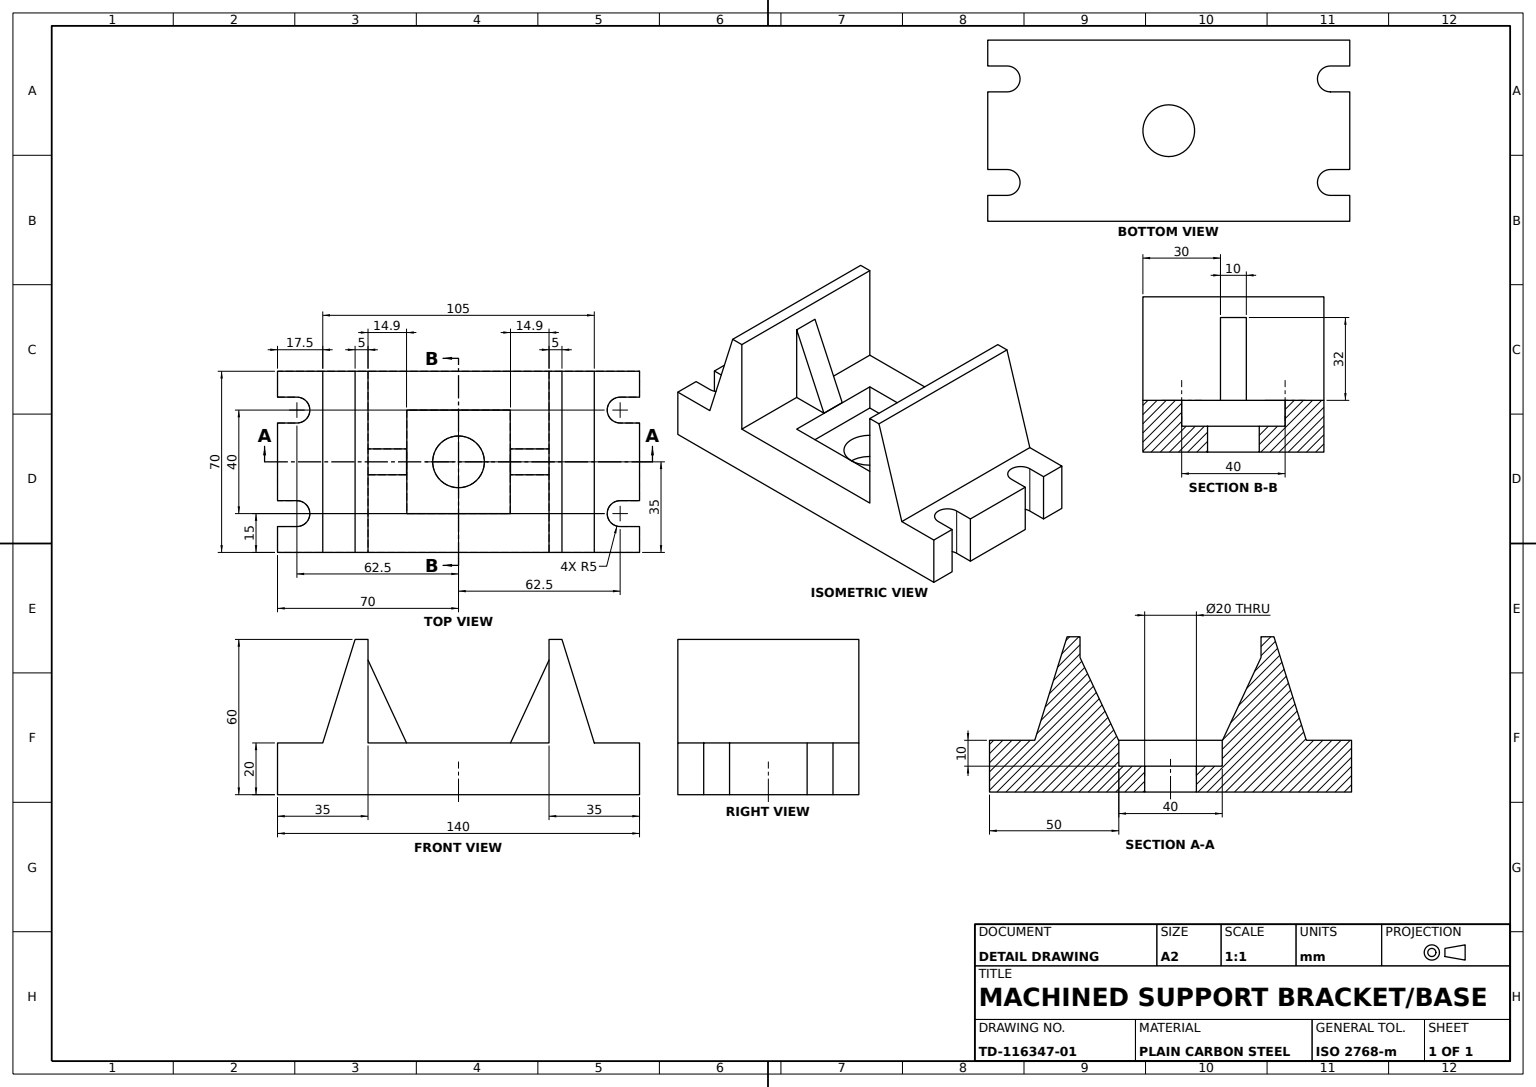
ISO-10303-21;
HEADER;
FILE_DESCRIPTION((''),'2;1');
FILE_NAME('','',(''),(''),'','','');
FILE_SCHEMA(('AUTOMOTIVE_DESIGN'));
ENDSEC;
DATA;
#1=APPLICATION_CONTEXT('');
#2=PRODUCT_CONTEXT('',#1,'mechanical');
#3=PRODUCT('','','',(#2));
#4=PRODUCT_DEFINITION_FORMATION('','',#3);
#5=PRODUCT_DEFINITION_CONTEXT('',#1,'design');
#6=PRODUCT_DEFINITION('','',#4,#5);
#7=PRODUCT_DEFINITION_SHAPE('','',#6);
#8=(LENGTH_UNIT()NAMED_UNIT(*)SI_UNIT(.MILLI.,.METRE.));
#9=(NAMED_UNIT(*)PLANE_ANGLE_UNIT()SI_UNIT($,.RADIAN.));
#10=(NAMED_UNIT(*)SI_UNIT($,.STERADIAN.)SOLID_ANGLE_UNIT());
#11=UNCERTAINTY_MEASURE_WITH_UNIT(LENGTH_MEASURE(1.E-05),#8,'distance_accuracy_value','');
#12=(GEOMETRIC_REPRESENTATION_CONTEXT(3)GLOBAL_UNCERTAINTY_ASSIGNED_CONTEXT((#11))GLOBAL_UNIT_ASSIGNED_CONTEXT((#8,#9,#10))REPRESENTATION_CONTEXT('',''));
#13=CARTESIAN_POINT('',(-20.,10.,-20.));
#14=VERTEX_POINT('',#13);
#15=CARTESIAN_POINT('',(-20.,10.,20.));
#16=VERTEX_POINT('',#15);
#17=DIRECTION('',(0.,0.,1.));
#18=VECTOR('',#17,1000.);
#19=LINE('',#13,#18);
#20=EDGE_CURVE('',#14,#16,#19,.T.);
#21=ORIENTED_EDGE('',*,*,#20,.F.);
#22=CARTESIAN_POINT('',(-20.,20.,-20.));
#23=VERTEX_POINT('',#22);
#24=DIRECTION('',(0.,1.,0.));
#25=VECTOR('',#24,1000.);
#26=LINE('',#13,#25);
#27=EDGE_CURVE('',#14,#23,#26,.T.);
#28=ORIENTED_EDGE('',*,*,#27,.T.);
#29=CARTESIAN_POINT('',(-20.,20.,20.));
#30=VERTEX_POINT('',#29);
#31=LINE('',#22,#18);
#32=EDGE_CURVE('',#23,#30,#31,.T.);
#33=ORIENTED_EDGE('',*,*,#32,.T.);
#34=LINE('',#15,#25);
#35=EDGE_CURVE('',#16,#30,#34,.T.);
#36=ORIENTED_EDGE('',*,*,#35,.F.);
#37=EDGE_LOOP('',(#21,#28,#33,#36));
#38=FACE_OUTER_BOUND('',#37,.T.);
#39=DIRECTION('',(-1.,0.,0.));
#40=AXIS2_PLACEMENT_3D('',#13,#39,#17);
#41=PLANE('',#40);
#42=ADVANCED_FACE('',(#38),#41,.F.);
#43=CARTESIAN_POINT('',(70.,20.,15.));
#44=VERTEX_POINT('',#43);
#45=CARTESIAN_POINT('',(70.,0.,15.));
#46=VERTEX_POINT('',#45);
#47=DIRECTION('',(0.,-1.,0.));
#48=VECTOR('',#47,1000.);
#49=LINE('',#43,#48);
#50=EDGE_CURVE('',#44,#46,#49,.T.);
#51=ORIENTED_EDGE('',*,*,#50,.T.);
#52=CARTESIAN_POINT('',(70.,0.,-15.));
#53=VERTEX_POINT('',#52);
#54=DIRECTION('',(0.,0.,-1.));
#55=VECTOR('',#54,1000.);
#56=LINE('',#52,#55);
#57=EDGE_CURVE('',#46,#53,#56,.T.);
#58=ORIENTED_EDGE('',*,*,#57,.T.);
#59=CARTESIAN_POINT('',(70.,20.,-15.));
#60=VERTEX_POINT('',#59);
#61=LINE('',#59,#48);
#62=EDGE_CURVE('',#60,#53,#61,.T.);
#63=ORIENTED_EDGE('',*,*,#62,.F.);
#64=LINE('',#59,#55);
#65=EDGE_CURVE('',#44,#60,#64,.T.);
#66=ORIENTED_EDGE('',*,*,#65,.F.);
#67=EDGE_LOOP('',(#51,#58,#63,#66));
#68=FACE_OUTER_BOUND('',#67,.T.);
#69=AXIS2_PLACEMENT_3D('',#59,#39,#17);
#70=PLANE('',#69);
#71=ADVANCED_FACE('',(#68),#70,.F.);
#72=ORIENTED_EDGE('',*,*,#35,.T.);
#73=CARTESIAN_POINT('',(20.,20.,20.));
#74=VERTEX_POINT('',#73);
#75=DIRECTION('',(1.,0.,0.));
#76=VECTOR('',#75,1000.);
#77=LINE('',#29,#76);
#78=EDGE_CURVE('',#30,#74,#77,.T.);
#79=ORIENTED_EDGE('',*,*,#78,.T.);
#80=CARTESIAN_POINT('',(20.,10.,20.));
#81=VERTEX_POINT('',#80);
#82=LINE('',#80,#25);
#83=EDGE_CURVE('',#81,#74,#82,.T.);
#84=ORIENTED_EDGE('',*,*,#83,.F.);
#85=LINE('',#15,#76);
#86=EDGE_CURVE('',#16,#81,#85,.T.);
#87=ORIENTED_EDGE('',*,*,#86,.F.);
#88=EDGE_LOOP('',(#72,#79,#84,#87));
#89=FACE_OUTER_BOUND('',#88,.T.);
#90=AXIS2_PLACEMENT_3D('',#15,#17,#75);
#91=PLANE('',#90);
#92=ADVANCED_FACE('',(#89),#91,.F.);
#93=CARTESIAN_POINT('',(62.5,0.,-25.));
#94=VERTEX_POINT('',#93);
#95=CARTESIAN_POINT('',(70.,0.,-25.));
#96=VERTEX_POINT('',#95);
#97=LINE('',#93,#76);
#98=EDGE_CURVE('',#94,#96,#97,.T.);
#99=ORIENTED_EDGE('',*,*,#98,.T.);
#100=CARTESIAN_POINT('',(70.,20.,-25.));
#101=VERTEX_POINT('',#100);
#102=LINE('',#100,#48);
#103=EDGE_CURVE('',#101,#96,#102,.T.);
#104=ORIENTED_EDGE('',*,*,#103,.F.);
#105=CARTESIAN_POINT('',(62.5,20.,-25.));
#106=VERTEX_POINT('',#105);
#107=LINE('',#105,#76);
#108=EDGE_CURVE('',#106,#101,#107,.T.);
#109=ORIENTED_EDGE('',*,*,#108,.F.);
#110=LINE('',#105,#48);
#111=EDGE_CURVE('',#106,#94,#110,.T.);
#112=ORIENTED_EDGE('',*,*,#111,.T.);
#113=EDGE_LOOP('',(#99,#104,#109,#112));
#114=FACE_OUTER_BOUND('',#113,.T.);
#115=AXIS2_PLACEMENT_3D('',#105,#54,#39);
#116=PLANE('',#115);
#117=ADVANCED_FACE('',(#114),#116,.F.);
#118=CARTESIAN_POINT('',(62.5,0.,25.));
#119=VERTEX_POINT('',#118);
#120=CARTESIAN_POINT('',(62.5,0.,15.));
#121=VERTEX_POINT('',#120);
#122=CARTESIAN_POINT('',(62.5,0.,20.));
#123=AXIS2_PLACEMENT_3D('',#122,#47,#17);
#124=CIRCLE('',#123,5.);
#125=EDGE_CURVE('',#119,#121,#124,.T.);
#126=ORIENTED_EDGE('',*,*,#125,.T.);
#127=CARTESIAN_POINT('',(62.5,20.,15.));
#128=VERTEX_POINT('',#127);
#129=LINE('',#127,#48);
#130=EDGE_CURVE('',#128,#121,#129,.T.);
#131=ORIENTED_EDGE('',*,*,#130,.F.);
#132=CARTESIAN_POINT('',(62.5,20.,25.));
#133=VERTEX_POINT('',#132);
#134=CARTESIAN_POINT('',(62.5,20.,20.));
#135=AXIS2_PLACEMENT_3D('',#134,#47,#17);
#136=CIRCLE('',#135,5.);
#137=EDGE_CURVE('',#133,#128,#136,.T.);
#138=ORIENTED_EDGE('',*,*,#137,.F.);
#139=LINE('',#132,#48);
#140=EDGE_CURVE('',#133,#119,#139,.T.);
#141=ORIENTED_EDGE('',*,*,#140,.T.);
#142=EDGE_LOOP('',(#126,#131,#138,#141));
#143=FACE_OUTER_BOUND('',#142,.T.);
#144=AXIS2_PLACEMENT_3D('',#134,#47,#54);
#145=CYLINDRICAL_SURFACE('',#144,5.);
#146=ADVANCED_FACE('',(#143),#145,.F.);
#147=CARTESIAN_POINT('',(70.,0.,25.));
#148=VERTEX_POINT('',#147);
#149=VECTOR('',#39,1000.);
#150=LINE('',#147,#149);
#151=EDGE_CURVE('',#148,#119,#150,.T.);
#152=ORIENTED_EDGE('',*,*,#151,.T.);
#153=ORIENTED_EDGE('',*,*,#140,.F.);
#154=CARTESIAN_POINT('',(70.,20.,25.));
#155=VERTEX_POINT('',#154);
#156=LINE('',#154,#149);
#157=EDGE_CURVE('',#155,#133,#156,.T.);
#158=ORIENTED_EDGE('',*,*,#157,.F.);
#159=LINE('',#154,#48);
#160=EDGE_CURVE('',#155,#148,#159,.T.);
#161=ORIENTED_EDGE('',*,*,#160,.T.);
#162=EDGE_LOOP('',(#152,#153,#158,#161));
#163=FACE_OUTER_BOUND('',#162,.T.);
#164=AXIS2_PLACEMENT_3D('',#154,#17,#75);
#165=PLANE('',#164);
#166=ADVANCED_FACE('',(#163),#165,.F.);
#167=CARTESIAN_POINT('',(20.1,20.,-5.));
#168=VERTEX_POINT('',#167);
#169=CARTESIAN_POINT('',(35.,52.,-5.));
#170=VERTEX_POINT('',#169);
#171=CARTESIAN_POINT('',(8.865418,-4.12796,-5.));
#172=DIRECTION('',(0.422109867,0.906544682,0.));
#173=VECTOR('',#172,1000.);
#174=LINE('',#171,#173);
#175=EDGE_CURVE('',#168,#170,#174,.T.);
#176=ORIENTED_EDGE('',*,*,#175,.T.);
#177=CARTESIAN_POINT('',(35.,20.,-5.));
#178=VERTEX_POINT('',#177);
#179=CARTESIAN_POINT('',(35.,0.,-5.));
#180=LINE('',#179,#48);
#181=EDGE_CURVE('',#170,#178,#180,.T.);
#182=ORIENTED_EDGE('',*,*,#181,.T.);
#183=CARTESIAN_POINT('',(0.,20.,-5.));
#184=LINE('',#183,#149);
#185=EDGE_CURVE('',#178,#168,#184,.T.);
#186=ORIENTED_EDGE('',*,*,#185,.T.);
#187=EDGE_LOOP('',(#176,#182,#186));
#188=FACE_OUTER_BOUND('',#187,.T.);
#189=CARTESIAN_POINT('',(0.,0.,-5.));
#190=AXIS2_PLACEMENT_3D('',#189,#17,#75);
#191=PLANE('',#190);
#192=ADVANCED_FACE('',(#188),#191,.F.);
#193=CARTESIAN_POINT('',(70.,20.,-35.));
#194=VERTEX_POINT('',#193);
#195=CARTESIAN_POINT('',(70.,0.,-35.));
#196=VERTEX_POINT('',#195);
#197=LINE('',#193,#48);
#198=EDGE_CURVE('',#194,#196,#197,.T.);
#199=ORIENTED_EDGE('',*,*,#198,.F.);
#200=LINE('',#193,#55);
#201=EDGE_CURVE('',#101,#194,#200,.T.);
#202=ORIENTED_EDGE('',*,*,#201,.F.);
#203=ORIENTED_EDGE('',*,*,#103,.T.);
#204=LINE('',#195,#55);
#205=EDGE_CURVE('',#96,#196,#204,.T.);
#206=ORIENTED_EDGE('',*,*,#205,.T.);
#207=EDGE_LOOP('',(#199,#202,#203,#206));
#208=FACE_OUTER_BOUND('',#207,.T.);
#209=AXIS2_PLACEMENT_3D('',#193,#39,#17);
#210=PLANE('',#209);
#211=ADVANCED_FACE('',(#208),#210,.F.);
#212=ORIENTED_EDGE('',*,*,#130,.T.);
#213=LINE('',#120,#76);
#214=EDGE_CURVE('',#121,#46,#213,.T.);
#215=ORIENTED_EDGE('',*,*,#214,.T.);
#216=ORIENTED_EDGE('',*,*,#50,.F.);
#217=LINE('',#127,#76);
#218=EDGE_CURVE('',#128,#44,#217,.T.);
#219=ORIENTED_EDGE('',*,*,#218,.F.);
#220=EDGE_LOOP('',(#212,#215,#216,#219));
#221=FACE_OUTER_BOUND('',#220,.T.);
#222=AXIS2_PLACEMENT_3D('',#127,#54,#39);
#223=PLANE('',#222);
#224=ADVANCED_FACE('',(#221),#223,.F.);
#225=CARTESIAN_POINT('',(-70.,20.,-35.));
#226=VERTEX_POINT('',#225);
#227=CARTESIAN_POINT('',(-70.,0.,-35.));
#228=VERTEX_POINT('',#227);
#229=LINE('',#225,#48);
#230=EDGE_CURVE('',#226,#228,#229,.T.);
#231=ORIENTED_EDGE('',*,*,#230,.F.);
#232=CARTESIAN_POINT('',(-52.5,20.,-35.));
#233=VERTEX_POINT('',#232);
#234=LINE('',#225,#149);
#235=EDGE_CURVE('',#233,#226,#234,.T.);
#236=ORIENTED_EDGE('',*,*,#235,.F.);
#237=CARTESIAN_POINT('',(-40.,60.,-35.));
#238=VERTEX_POINT('',#237);
#239=CARTESIAN_POINT('',(-53.523132,16.725979,-35.));
#240=DIRECTION('',(-0.298274993,-0.954479978,0.));
#241=VECTOR('',#240,1000.);
#242=LINE('',#239,#241);
#243=EDGE_CURVE('',#238,#233,#242,.T.);
#244=ORIENTED_EDGE('',*,*,#243,.F.);
#245=CARTESIAN_POINT('',(-35.,60.,-35.));
#246=VERTEX_POINT('',#245);
#247=CARTESIAN_POINT('',(0.,60.,-35.));
#248=LINE('',#247,#149);
#249=EDGE_CURVE('',#246,#238,#248,.T.);
#250=ORIENTED_EDGE('',*,*,#249,.F.);
#251=CARTESIAN_POINT('',(-35.,20.,-35.));
#252=VERTEX_POINT('',#251);
#253=CARTESIAN_POINT('',(-35.,0.,-35.));
#254=LINE('',#253,#25);
#255=EDGE_CURVE('',#252,#246,#254,.T.);
#256=ORIENTED_EDGE('',*,*,#255,.F.);
#257=CARTESIAN_POINT('',(35.,20.,-35.));
#258=VERTEX_POINT('',#257);
#259=EDGE_CURVE('',#258,#252,#234,.T.);
#260=ORIENTED_EDGE('',*,*,#259,.F.);
#261=CARTESIAN_POINT('',(35.,60.,-35.));
#262=VERTEX_POINT('',#261);
#263=CARTESIAN_POINT('',(35.,0.,-35.));
#264=LINE('',#263,#48);
#265=EDGE_CURVE('',#262,#258,#264,.T.);
#266=ORIENTED_EDGE('',*,*,#265,.F.);
#267=CARTESIAN_POINT('',(40.,60.,-35.));
#268=VERTEX_POINT('',#267);
#269=LINE('',#247,#76);
#270=EDGE_CURVE('',#262,#268,#269,.T.);
#271=ORIENTED_EDGE('',*,*,#270,.T.);
#272=CARTESIAN_POINT('',(52.5,20.,-35.));
#273=VERTEX_POINT('',#272);
#274=CARTESIAN_POINT('',(53.523132,16.725979,-35.));
#275=DIRECTION('',(0.298274993,-0.954479978,0.));
#276=VECTOR('',#275,1000.);
#277=LINE('',#274,#276);
#278=EDGE_CURVE('',#268,#273,#277,.T.);
#279=ORIENTED_EDGE('',*,*,#278,.T.);
#280=EDGE_CURVE('',#194,#273,#234,.T.);
#281=ORIENTED_EDGE('',*,*,#280,.F.);
#282=ORIENTED_EDGE('',*,*,#198,.T.);
#283=LINE('',#227,#149);
#284=EDGE_CURVE('',#196,#228,#283,.T.);
#285=ORIENTED_EDGE('',*,*,#284,.T.);
#286=EDGE_LOOP('',(#231,#236,#244,#250,#256,#260,#266,#271,#279,#281,#282,#285));
#287=FACE_OUTER_BOUND('',#286,.T.);
#288=AXIS2_PLACEMENT_3D('',#225,#17,#75);
#289=PLANE('',#288);
#290=ADVANCED_FACE('',(#287),#289,.F.);
#291=CARTESIAN_POINT('',(0.,0.,-10.));
#292=VERTEX_POINT('',#291);
#293=CARTESIAN_POINT('',(0.,0.,10.));
#294=VERTEX_POINT('',#293);
#295=CARTESIAN_POINT('',(0.,0.,0.));
#296=AXIS2_PLACEMENT_3D('',#295,#24,#17);
#297=CIRCLE('',#296,10.);
#298=EDGE_CURVE('',#292,#294,#297,.T.);
#299=ORIENTED_EDGE('',*,*,#298,.F.);
#300=CARTESIAN_POINT('',(0.,10.,-10.));
#301=VERTEX_POINT('',#300);
#302=LINE('',#291,#25);
#303=EDGE_CURVE('',#292,#301,#302,.T.);
#304=ORIENTED_EDGE('',*,*,#303,.T.);
#305=CARTESIAN_POINT('',(0.,10.,10.));
#306=VERTEX_POINT('',#305);
#307=CARTESIAN_POINT('',(0.,10.,0.));
#308=AXIS2_PLACEMENT_3D('',#307,#47,#17);
#309=CIRCLE('',#308,10.);
#310=EDGE_CURVE('',#306,#301,#309,.T.);
#311=ORIENTED_EDGE('',*,*,#310,.F.);
#312=LINE('',#293,#25);
#313=EDGE_CURVE('',#294,#306,#312,.T.);
#314=ORIENTED_EDGE('',*,*,#313,.F.);
#315=EDGE_LOOP('',(#299,#304,#311,#314));
#316=FACE_OUTER_BOUND('',#315,.T.);
#317=CYLINDRICAL_SURFACE('',#296,10.);
#318=ADVANCED_FACE('',(#316),#317,.F.);
#319=ORIENTED_EDGE('',*,*,#249,.T.);
#320=CARTESIAN_POINT('',(-40.,60.,35.));
#321=VERTEX_POINT('',#320);
#322=LINE('',#237,#18);
#323=EDGE_CURVE('',#238,#321,#322,.T.);
#324=ORIENTED_EDGE('',*,*,#323,.T.);
#325=CARTESIAN_POINT('',(-35.,60.,35.));
#326=VERTEX_POINT('',#325);
#327=CARTESIAN_POINT('',(0.,60.,35.));
#328=LINE('',#327,#149);
#329=EDGE_CURVE('',#326,#321,#328,.T.);
#330=ORIENTED_EDGE('',*,*,#329,.F.);
#331=LINE('',#245,#18);
#332=EDGE_CURVE('',#246,#326,#331,.T.);
#333=ORIENTED_EDGE('',*,*,#332,.F.);
#334=EDGE_LOOP('',(#319,#324,#330,#333));
#335=FACE_OUTER_BOUND('',#334,.T.);
#336=AXIS2_PLACEMENT_3D('',#247,#24,#17);
#337=PLANE('',#336);
#338=ADVANCED_FACE('',(#335),#337,.T.);
#339=CARTESIAN_POINT('',(35.,60.,35.));
#340=VERTEX_POINT('',#339);
#341=LINE('',#261,#18);
#342=EDGE_CURVE('',#262,#340,#341,.T.);
#343=ORIENTED_EDGE('',*,*,#342,.T.);
#344=CARTESIAN_POINT('',(40.,60.,35.));
#345=VERTEX_POINT('',#344);
#346=LINE('',#327,#76);
#347=EDGE_CURVE('',#340,#345,#346,.T.);
#348=ORIENTED_EDGE('',*,*,#347,.T.);
#349=LINE('',#267,#18);
#350=EDGE_CURVE('',#268,#345,#349,.T.);
#351=ORIENTED_EDGE('',*,*,#350,.F.);
#352=ORIENTED_EDGE('',*,*,#270,.F.);
#353=EDGE_LOOP('',(#343,#348,#351,#352));
#354=FACE_OUTER_BOUND('',#353,.T.);
#355=AXIS2_PLACEMENT_3D('',#247,#47,#54);
#356=PLANE('',#355);
#357=ADVANCED_FACE('',(#354),#356,.F.);
#358=ORIENTED_EDGE('',*,*,#78,.F.);
#359=ORIENTED_EDGE('',*,*,#32,.F.);
#360=CARTESIAN_POINT('',(20.,20.,-20.));
#361=VERTEX_POINT('',#360);
#362=LINE('',#22,#149);
#363=EDGE_CURVE('',#361,#23,#362,.T.);
#364=ORIENTED_EDGE('',*,*,#363,.F.);
#365=LINE('',#360,#55);
#366=EDGE_CURVE('',#74,#361,#365,.T.);
#367=ORIENTED_EDGE('',*,*,#366,.F.);
#368=EDGE_LOOP('',(#358,#359,#364,#367));
#369=FACE_BOUND('',#368,.T.);
#370=CARTESIAN_POINT('',(-35.,20.,-5.));
#371=VERTEX_POINT('',#370);
#372=LINE('',#251,#18);
#373=EDGE_CURVE('',#252,#371,#372,.T.);
#374=ORIENTED_EDGE('',*,*,#373,.T.);
#375=CARTESIAN_POINT('',(-20.102952,20.,-5.));
#376=VERTEX_POINT('',#375);
#377=EDGE_CURVE('',#376,#371,#184,.T.);
#378=ORIENTED_EDGE('',*,*,#377,.F.);
#379=CARTESIAN_POINT('',(-20.102952,20.,5.));
#380=VERTEX_POINT('',#379);
#381=LINE('',#379,#55);
#382=EDGE_CURVE('',#380,#376,#381,.T.);
#383=ORIENTED_EDGE('',*,*,#382,.F.);
#384=CARTESIAN_POINT('',(-35.,20.,5.));
#385=VERTEX_POINT('',#384);
#386=CARTESIAN_POINT('',(0.,20.,5.));
#387=LINE('',#386,#149);
#388=EDGE_CURVE('',#380,#385,#387,.T.);
#389=ORIENTED_EDGE('',*,*,#388,.T.);
#390=CARTESIAN_POINT('',(-35.,20.,35.));
#391=VERTEX_POINT('',#390);
#392=EDGE_CURVE('',#385,#391,#372,.T.);
#393=ORIENTED_EDGE('',*,*,#392,.T.);
#394=CARTESIAN_POINT('',(35.,20.,35.));
#395=VERTEX_POINT('',#394);
#396=CARTESIAN_POINT('',(-70.,20.,35.));
#397=LINE('',#396,#76);
#398=EDGE_CURVE('',#391,#395,#397,.T.);
#399=ORIENTED_EDGE('',*,*,#398,.T.);
#400=CARTESIAN_POINT('',(35.,20.,5.));
#401=VERTEX_POINT('',#400);
#402=LINE('',#257,#18);
#403=EDGE_CURVE('',#401,#395,#402,.T.);
#404=ORIENTED_EDGE('',*,*,#403,.F.);
#405=CARTESIAN_POINT('',(20.1,20.,5.));
#406=VERTEX_POINT('',#405);
#407=EDGE_CURVE('',#401,#406,#387,.T.);
#408=ORIENTED_EDGE('',*,*,#407,.T.);
#409=LINE('',#405,#55);
#410=EDGE_CURVE('',#406,#168,#409,.T.);
#411=ORIENTED_EDGE('',*,*,#410,.T.);
#412=ORIENTED_EDGE('',*,*,#185,.F.);
#413=EDGE_CURVE('',#258,#178,#402,.T.);
#414=ORIENTED_EDGE('',*,*,#413,.F.);
#415=ORIENTED_EDGE('',*,*,#259,.T.);
#416=EDGE_LOOP('',(#374,#378,#383,#389,#393,#399,#404,#408,#411,#412,#414,#415));
#417=FACE_OUTER_BOUND('',#416,.T.);
#418=CARTESIAN_POINT('',(62.5,20.,-20.));
#419=AXIS2_PLACEMENT_3D('',#418,#24,#17);
#420=PLANE('',#419);
#421=ADVANCED_FACE('',(#369,#417),#420,.T.);
#422=CARTESIAN_POINT('',(62.5,20.,-15.));
#423=VERTEX_POINT('',#422);
#424=AXIS2_PLACEMENT_3D('',#418,#47,#17);
#425=CIRCLE('',#424,5.);
#426=EDGE_CURVE('',#423,#106,#425,.T.);
#427=ORIENTED_EDGE('',*,*,#426,.F.);
#428=CARTESIAN_POINT('',(62.5,0.,-15.));
#429=VERTEX_POINT('',#428);
#430=LINE('',#422,#48);
#431=EDGE_CURVE('',#423,#429,#430,.T.);
#432=ORIENTED_EDGE('',*,*,#431,.T.);
#433=CARTESIAN_POINT('',(62.5,0.,-20.));
#434=AXIS2_PLACEMENT_3D('',#433,#47,#17);
#435=CIRCLE('',#434,5.);
#436=EDGE_CURVE('',#429,#94,#435,.T.);
#437=ORIENTED_EDGE('',*,*,#436,.T.);
#438=ORIENTED_EDGE('',*,*,#111,.F.);
#439=EDGE_LOOP('',(#427,#432,#437,#438));
#440=FACE_OUTER_BOUND('',#439,.T.);
#441=AXIS2_PLACEMENT_3D('',#418,#47,#54);
#442=CYLINDRICAL_SURFACE('',#441,5.);
#443=ADVANCED_FACE('',(#440),#442,.F.);
#444=CARTESIAN_POINT('',(-62.5,0.,-15.));
#445=VERTEX_POINT('',#444);
#446=CARTESIAN_POINT('',(-70.,0.,-15.));
#447=VERTEX_POINT('',#446);
#448=LINE('',#444,#149);
#449=EDGE_CURVE('',#445,#447,#448,.T.);
#450=ORIENTED_EDGE('',*,*,#449,.T.);
#451=CARTESIAN_POINT('',(-70.,20.,-15.));
#452=VERTEX_POINT('',#451);
#453=LINE('',#451,#48);
#454=EDGE_CURVE('',#452,#447,#453,.T.);
#455=ORIENTED_EDGE('',*,*,#454,.F.);
#456=CARTESIAN_POINT('',(-62.5,20.,-15.));
#457=VERTEX_POINT('',#456);
#458=LINE('',#456,#149);
#459=EDGE_CURVE('',#457,#452,#458,.T.);
#460=ORIENTED_EDGE('',*,*,#459,.F.);
#461=LINE('',#456,#48);
#462=EDGE_CURVE('',#457,#445,#461,.T.);
#463=ORIENTED_EDGE('',*,*,#462,.T.);
#464=EDGE_LOOP('',(#450,#455,#460,#463));
#465=FACE_OUTER_BOUND('',#464,.T.);
#466=AXIS2_PLACEMENT_3D('',#456,#17,#75);
#467=PLANE('',#466);
#468=ADVANCED_FACE('',(#465),#467,.F.);
#469=CARTESIAN_POINT('',(20.,10.,-20.));
#470=VERTEX_POINT('',#469);
#471=LINE('',#469,#25);
#472=EDGE_CURVE('',#470,#361,#471,.T.);
#473=ORIENTED_EDGE('',*,*,#472,.F.);
#474=LINE('',#469,#55);
#475=EDGE_CURVE('',#81,#470,#474,.T.);
#476=ORIENTED_EDGE('',*,*,#475,.F.);
#477=ORIENTED_EDGE('',*,*,#83,.T.);
#478=ORIENTED_EDGE('',*,*,#366,.T.);
#479=EDGE_LOOP('',(#473,#476,#477,#478));
#480=FACE_OUTER_BOUND('',#479,.T.);
#481=AXIS2_PLACEMENT_3D('',#469,#75,#54);
#482=PLANE('',#481);
#483=ADVANCED_FACE('',(#480),#482,.F.);
#484=CARTESIAN_POINT('',(-35.,52.,5.));
#485=VERTEX_POINT('',#484);
#486=CARTESIAN_POINT('',(-35.,52.,-5.));
#487=VERTEX_POINT('',#486);
#488=LINE('',#484,#55);
#489=EDGE_CURVE('',#485,#487,#488,.T.);
#490=ORIENTED_EDGE('',*,*,#489,.F.);
#491=CARTESIAN_POINT('',(-8.869987,-4.129269,5.));
#492=DIRECTION('',(0.422041138,-0.906576681,0.));
#493=VECTOR('',#492,1000.);
#494=LINE('',#491,#493);
#495=EDGE_CURVE('',#485,#380,#494,.T.);
#496=ORIENTED_EDGE('',*,*,#495,.T.);
#497=ORIENTED_EDGE('',*,*,#382,.T.);
#498=CARTESIAN_POINT('',(-8.869987,-4.129269,-5.));
#499=LINE('',#498,#493);
#500=EDGE_CURVE('',#487,#376,#499,.T.);
#501=ORIENTED_EDGE('',*,*,#500,.F.);
#502=EDGE_LOOP('',(#490,#496,#497,#501));
#503=FACE_OUTER_BOUND('',#502,.T.);
#504=DIRECTION('',(0.906576681,0.422041138,0.));
#505=DIRECTION('',(-0.422041138,0.906576681,0.));
#506=AXIS2_PLACEMENT_3D('',#491,#504,#505);
#507=PLANE('',#506);
#508=ADVANCED_FACE('',(#503),#507,.T.);
#509=CARTESIAN_POINT('',(-70.,20.,25.));
#510=VERTEX_POINT('',#509);
#511=VERTEX_POINT('',#396);
#512=LINE('',#509,#18);
#513=EDGE_CURVE('',#510,#511,#512,.T.);
#514=ORIENTED_EDGE('',*,*,#513,.T.);
#515=CARTESIAN_POINT('',(-52.5,20.,35.));
#516=VERTEX_POINT('',#515);
#517=EDGE_CURVE('',#511,#516,#397,.T.);
#518=ORIENTED_EDGE('',*,*,#517,.T.);
#519=LINE('',#232,#18);
#520=EDGE_CURVE('',#233,#516,#519,.T.);
#521=ORIENTED_EDGE('',*,*,#520,.F.);
#522=ORIENTED_EDGE('',*,*,#235,.T.);
#523=CARTESIAN_POINT('',(-70.,20.,-25.));
#524=VERTEX_POINT('',#523);
#525=LINE('',#225,#18);
#526=EDGE_CURVE('',#226,#524,#525,.T.);
#527=ORIENTED_EDGE('',*,*,#526,.T.);
#528=CARTESIAN_POINT('',(-62.5,20.,-25.));
#529=VERTEX_POINT('',#528);
#530=LINE('',#523,#76);
#531=EDGE_CURVE('',#524,#529,#530,.T.);
#532=ORIENTED_EDGE('',*,*,#531,.T.);
#533=CARTESIAN_POINT('',(-62.5,20.,-20.));
#534=AXIS2_PLACEMENT_3D('',#533,#47,#17);
#535=CIRCLE('',#534,5.);
#536=EDGE_CURVE('',#529,#457,#535,.T.);
#537=ORIENTED_EDGE('',*,*,#536,.T.);
#538=ORIENTED_EDGE('',*,*,#459,.T.);
#539=CARTESIAN_POINT('',(-70.,20.,15.));
#540=VERTEX_POINT('',#539);
#541=LINE('',#451,#18);
#542=EDGE_CURVE('',#452,#540,#541,.T.);
#543=ORIENTED_EDGE('',*,*,#542,.T.);
#544=CARTESIAN_POINT('',(-62.5,20.,15.));
#545=VERTEX_POINT('',#544);
#546=LINE('',#539,#76);
#547=EDGE_CURVE('',#540,#545,#546,.T.);
#548=ORIENTED_EDGE('',*,*,#547,.T.);
#549=CARTESIAN_POINT('',(-62.5,20.,25.));
#550=VERTEX_POINT('',#549);
#551=CARTESIAN_POINT('',(-62.5,20.,20.));
#552=AXIS2_PLACEMENT_3D('',#551,#47,#17);
#553=CIRCLE('',#552,5.);
#554=EDGE_CURVE('',#545,#550,#553,.T.);
#555=ORIENTED_EDGE('',*,*,#554,.T.);
#556=LINE('',#549,#149);
#557=EDGE_CURVE('',#550,#510,#556,.T.);
#558=ORIENTED_EDGE('',*,*,#557,.T.);
#559=EDGE_LOOP('',(#514,#518,#521,#522,#527,#532,#537,#538,#543,#548,#555,#558));
#560=FACE_OUTER_BOUND('',#559,.T.);
#561=ADVANCED_FACE('',(#560),#420,.T.);
#562=CARTESIAN_POINT('',(35.,52.,5.));
#563=VERTEX_POINT('',#562);
#564=CARTESIAN_POINT('',(35.,0.,5.));
#565=LINE('',#564,#48);
#566=EDGE_CURVE('',#563,#401,#565,.T.);
#567=ORIENTED_EDGE('',*,*,#566,.F.);
#568=CARTESIAN_POINT('',(8.865418,-4.12796,5.));
#569=LINE('',#568,#173);
#570=EDGE_CURVE('',#406,#563,#569,.T.);
#571=ORIENTED_EDGE('',*,*,#570,.F.);
#572=ORIENTED_EDGE('',*,*,#407,.F.);
#573=EDGE_LOOP('',(#567,#571,#572));
#574=FACE_OUTER_BOUND('',#573,.T.);
#575=CARTESIAN_POINT('',(0.,0.,5.));
#576=AXIS2_PLACEMENT_3D('',#575,#17,#75);
#577=PLANE('',#576);
#578=ADVANCED_FACE('',(#574),#577,.T.);
#579=CARTESIAN_POINT('',(70.,20.,35.));
#580=VERTEX_POINT('',#579);
#581=LINE('',#154,#55);
#582=EDGE_CURVE('',#580,#155,#581,.T.);
#583=ORIENTED_EDGE('',*,*,#582,.T.);
#584=ORIENTED_EDGE('',*,*,#157,.T.);
#585=ORIENTED_EDGE('',*,*,#137,.T.);
#586=ORIENTED_EDGE('',*,*,#218,.T.);
#587=ORIENTED_EDGE('',*,*,#65,.T.);
#588=LINE('',#59,#149);
#589=EDGE_CURVE('',#60,#423,#588,.T.);
#590=ORIENTED_EDGE('',*,*,#589,.T.);
#591=ORIENTED_EDGE('',*,*,#426,.T.);
#592=ORIENTED_EDGE('',*,*,#108,.T.);
#593=ORIENTED_EDGE('',*,*,#201,.T.);
#594=ORIENTED_EDGE('',*,*,#280,.T.);
#595=CARTESIAN_POINT('',(52.5,20.,35.));
#596=VERTEX_POINT('',#595);
#597=LINE('',#272,#18);
#598=EDGE_CURVE('',#273,#596,#597,.T.);
#599=ORIENTED_EDGE('',*,*,#598,.T.);
#600=EDGE_CURVE('',#596,#580,#397,.T.);
#601=ORIENTED_EDGE('',*,*,#600,.T.);
#602=EDGE_LOOP('',(#583,#584,#585,#586,#587,#590,#591,#592,#593,#594,#599,#601));
#603=FACE_OUTER_BOUND('',#602,.T.);
#604=ADVANCED_FACE('',(#603),#420,.T.);
#605=CARTESIAN_POINT('',(-62.5,0.,15.));
#606=VERTEX_POINT('',#605);
#607=CARTESIAN_POINT('',(-62.5,0.,25.));
#608=VERTEX_POINT('',#607);
#609=CARTESIAN_POINT('',(-62.5,0.,20.));
#610=AXIS2_PLACEMENT_3D('',#609,#47,#17);
#611=CIRCLE('',#610,5.);
#612=EDGE_CURVE('',#606,#608,#611,.T.);
#613=ORIENTED_EDGE('',*,*,#612,.T.);
#614=LINE('',#549,#48);
#615=EDGE_CURVE('',#550,#608,#614,.T.);
#616=ORIENTED_EDGE('',*,*,#615,.F.);
#617=ORIENTED_EDGE('',*,*,#554,.F.);
#618=LINE('',#544,#48);
#619=EDGE_CURVE('',#545,#606,#618,.T.);
#620=ORIENTED_EDGE('',*,*,#619,.T.);
#621=EDGE_LOOP('',(#613,#616,#617,#620));
#622=FACE_OUTER_BOUND('',#621,.T.);
#623=AXIS2_PLACEMENT_3D('',#551,#47,#54);
#624=CYLINDRICAL_SURFACE('',#623,5.);
#625=ADVANCED_FACE('',(#622),#624,.F.);
#626=ORIENTED_EDGE('',*,*,#230,.T.);
#627=CARTESIAN_POINT('',(-70.,0.,-25.));
#628=VERTEX_POINT('',#627);
#629=LINE('',#227,#18);
#630=EDGE_CURVE('',#228,#628,#629,.T.);
#631=ORIENTED_EDGE('',*,*,#630,.T.);
#632=LINE('',#523,#48);
#633=EDGE_CURVE('',#524,#628,#632,.T.);
#634=ORIENTED_EDGE('',*,*,#633,.F.);
#635=ORIENTED_EDGE('',*,*,#526,.F.);
#636=EDGE_LOOP('',(#626,#631,#634,#635));
#637=FACE_OUTER_BOUND('',#636,.T.);
#638=AXIS2_PLACEMENT_3D('',#225,#75,#54);
#639=PLANE('',#638);
#640=ADVANCED_FACE('',(#637),#639,.F.);
#641=ORIENTED_EDGE('',*,*,#388,.F.);
#642=ORIENTED_EDGE('',*,*,#495,.F.);
#643=CARTESIAN_POINT('',(-35.,0.,5.));
#644=LINE('',#643,#25);
#645=EDGE_CURVE('',#385,#485,#644,.T.);
#646=ORIENTED_EDGE('',*,*,#645,.F.);
#647=EDGE_LOOP('',(#641,#642,#646));
#648=FACE_OUTER_BOUND('',#647,.T.);
#649=ADVANCED_FACE('',(#648),#577,.T.);
#650=ORIENTED_EDGE('',*,*,#377,.T.);
#651=CARTESIAN_POINT('',(-35.,0.,-5.));
#652=LINE('',#651,#25);
#653=EDGE_CURVE('',#371,#487,#652,.T.);
#654=ORIENTED_EDGE('',*,*,#653,.T.);
#655=ORIENTED_EDGE('',*,*,#500,.T.);
#656=EDGE_LOOP('',(#650,#654,#655));
#657=FACE_OUTER_BOUND('',#656,.T.);
#658=ADVANCED_FACE('',(#657),#191,.F.);
#659=ORIENTED_EDGE('',*,*,#298,.T.);
#660=EDGE_CURVE('',#294,#292,#297,.T.);
#661=ORIENTED_EDGE('',*,*,#660,.T.);
#662=EDGE_LOOP('',(#659,#661));
#663=FACE_BOUND('',#662,.T.);
#664=ORIENTED_EDGE('',*,*,#630,.F.);
#665=ORIENTED_EDGE('',*,*,#284,.F.);
#666=ORIENTED_EDGE('',*,*,#205,.F.);
#667=ORIENTED_EDGE('',*,*,#98,.F.);
#668=ORIENTED_EDGE('',*,*,#436,.F.);
#669=LINE('',#52,#149);
#670=EDGE_CURVE('',#53,#429,#669,.T.);
#671=ORIENTED_EDGE('',*,*,#670,.F.);
#672=ORIENTED_EDGE('',*,*,#57,.F.);
#673=ORIENTED_EDGE('',*,*,#214,.F.);
#674=ORIENTED_EDGE('',*,*,#125,.F.);
#675=ORIENTED_EDGE('',*,*,#151,.F.);
#676=CARTESIAN_POINT('',(70.,0.,35.));
#677=VERTEX_POINT('',#676);
#678=LINE('',#147,#55);
#679=EDGE_CURVE('',#677,#148,#678,.T.);
#680=ORIENTED_EDGE('',*,*,#679,.F.);
#681=CARTESIAN_POINT('',(-70.,0.,35.));
#682=VERTEX_POINT('',#681);
#683=LINE('',#681,#76);
#684=EDGE_CURVE('',#682,#677,#683,.T.);
#685=ORIENTED_EDGE('',*,*,#684,.F.);
#686=CARTESIAN_POINT('',(-70.,0.,25.));
#687=VERTEX_POINT('',#686);
#688=LINE('',#686,#18);
#689=EDGE_CURVE('',#687,#682,#688,.T.);
#690=ORIENTED_EDGE('',*,*,#689,.F.);
#691=LINE('',#607,#149);
#692=EDGE_CURVE('',#608,#687,#691,.T.);
#693=ORIENTED_EDGE('',*,*,#692,.F.);
#694=ORIENTED_EDGE('',*,*,#612,.F.);
#695=CARTESIAN_POINT('',(-70.,0.,15.));
#696=VERTEX_POINT('',#695);
#697=LINE('',#695,#76);
#698=EDGE_CURVE('',#696,#606,#697,.T.);
#699=ORIENTED_EDGE('',*,*,#698,.F.);
#700=LINE('',#446,#18);
#701=EDGE_CURVE('',#447,#696,#700,.T.);
#702=ORIENTED_EDGE('',*,*,#701,.F.);
#703=ORIENTED_EDGE('',*,*,#449,.F.);
#704=CARTESIAN_POINT('',(-62.5,0.,-25.));
#705=VERTEX_POINT('',#704);
#706=CARTESIAN_POINT('',(-62.5,0.,-20.));
#707=AXIS2_PLACEMENT_3D('',#706,#47,#17);
#708=CIRCLE('',#707,5.);
#709=EDGE_CURVE('',#705,#445,#708,.T.);
#710=ORIENTED_EDGE('',*,*,#709,.F.);
#711=LINE('',#627,#76);
#712=EDGE_CURVE('',#628,#705,#711,.T.);
#713=ORIENTED_EDGE('',*,*,#712,.F.);
#714=EDGE_LOOP('',(#664,#665,#666,#667,#668,#671,#672,#673,#674,#675,#680,#685,#690,#693,#694,#699,#702,#703,#710,#713));
#715=FACE_OUTER_BOUND('',#714,.T.);
#716=AXIS2_PLACEMENT_3D('',#433,#24,#17);
#717=PLANE('',#716);
#718=ADVANCED_FACE('',(#663,#715),#717,.F.);
#719=ORIENTED_EDGE('',*,*,#255,.T.);
#720=ORIENTED_EDGE('',*,*,#332,.T.);
#721=CARTESIAN_POINT('',(-35.,0.,35.));
#722=LINE('',#721,#25);
#723=EDGE_CURVE('',#391,#326,#722,.T.);
#724=ORIENTED_EDGE('',*,*,#723,.F.);
#725=ORIENTED_EDGE('',*,*,#392,.F.);
#726=ORIENTED_EDGE('',*,*,#645,.T.);
#727=ORIENTED_EDGE('',*,*,#489,.T.);
#728=ORIENTED_EDGE('',*,*,#653,.F.);
#729=ORIENTED_EDGE('',*,*,#373,.F.);
#730=EDGE_LOOP('',(#719,#720,#724,#725,#726,#727,#728,#729));
#731=FACE_OUTER_BOUND('',#730,.T.);
#732=AXIS2_PLACEMENT_3D('',#253,#75,#54);
#733=PLANE('',#732);
#734=ADVANCED_FACE('',(#731),#733,.T.);
#735=CARTESIAN_POINT('',(-53.523132,16.725979,35.));
#736=LINE('',#735,#241);
#737=EDGE_CURVE('',#321,#516,#736,.T.);
#738=ORIENTED_EDGE('',*,*,#737,.T.);
#739=ORIENTED_EDGE('',*,*,#517,.F.);
#740=LINE('',#396,#48);
#741=EDGE_CURVE('',#511,#682,#740,.T.);
#742=ORIENTED_EDGE('',*,*,#741,.T.);
#743=ORIENTED_EDGE('',*,*,#684,.T.);
#744=LINE('',#579,#48);
#745=EDGE_CURVE('',#580,#677,#744,.T.);
#746=ORIENTED_EDGE('',*,*,#745,.F.);
#747=ORIENTED_EDGE('',*,*,#600,.F.);
#748=CARTESIAN_POINT('',(53.523132,16.725979,35.));
#749=LINE('',#748,#276);
#750=EDGE_CURVE('',#345,#596,#749,.T.);
#751=ORIENTED_EDGE('',*,*,#750,.F.);
#752=ORIENTED_EDGE('',*,*,#347,.F.);
#753=CARTESIAN_POINT('',(35.,0.,35.));
#754=LINE('',#753,#48);
#755=EDGE_CURVE('',#340,#395,#754,.T.);
#756=ORIENTED_EDGE('',*,*,#755,.T.);
#757=ORIENTED_EDGE('',*,*,#398,.F.);
#758=ORIENTED_EDGE('',*,*,#723,.T.);
#759=ORIENTED_EDGE('',*,*,#329,.T.);
#760=EDGE_LOOP('',(#738,#739,#742,#743,#746,#747,#751,#752,#756,#757,#758,#759));
#761=FACE_OUTER_BOUND('',#760,.T.);
#762=AXIS2_PLACEMENT_3D('',#396,#54,#39);
#763=PLANE('',#762);
#764=ADVANCED_FACE('',(#761),#763,.F.);
#765=LINE('',#509,#48);
#766=EDGE_CURVE('',#510,#687,#765,.T.);
#767=ORIENTED_EDGE('',*,*,#766,.F.);
#768=ORIENTED_EDGE('',*,*,#557,.F.);
#769=ORIENTED_EDGE('',*,*,#615,.T.);
#770=ORIENTED_EDGE('',*,*,#692,.T.);
#771=EDGE_LOOP('',(#767,#768,#769,#770));
#772=FACE_OUTER_BOUND('',#771,.T.);
#773=AXIS2_PLACEMENT_3D('',#549,#17,#75);
#774=PLANE('',#773);
#775=ADVANCED_FACE('',(#772),#774,.F.);
#776=ORIENTED_EDGE('',*,*,#62,.T.);
#777=ORIENTED_EDGE('',*,*,#670,.T.);
#778=ORIENTED_EDGE('',*,*,#431,.F.);
#779=ORIENTED_EDGE('',*,*,#589,.F.);
#780=EDGE_LOOP('',(#776,#777,#778,#779));
#781=FACE_OUTER_BOUND('',#780,.T.);
#782=AXIS2_PLACEMENT_3D('',#59,#17,#75);
#783=PLANE('',#782);
#784=ADVANCED_FACE('',(#781),#783,.F.);
#785=ORIENTED_EDGE('',*,*,#750,.T.);
#786=ORIENTED_EDGE('',*,*,#598,.F.);
#787=ORIENTED_EDGE('',*,*,#278,.F.);
#788=ORIENTED_EDGE('',*,*,#350,.T.);
#789=EDGE_LOOP('',(#785,#786,#787,#788));
#790=FACE_OUTER_BOUND('',#789,.T.);
#791=DIRECTION('',(-0.954479978,-0.298274993,0.));
#792=AXIS2_PLACEMENT_3D('',#274,#791,#275);
#793=PLANE('',#792);
#794=ADVANCED_FACE('',(#790),#793,.F.);
#795=ORIENTED_EDGE('',*,*,#243,.T.);
#796=ORIENTED_EDGE('',*,*,#520,.T.);
#797=ORIENTED_EDGE('',*,*,#737,.F.);
#798=ORIENTED_EDGE('',*,*,#323,.F.);
#799=EDGE_LOOP('',(#795,#796,#797,#798));
#800=FACE_OUTER_BOUND('',#799,.T.);
#801=DIRECTION('',(-0.954479978,0.298274993,0.));
#802=AXIS2_PLACEMENT_3D('',#239,#801,#240);
#803=PLANE('',#802);
#804=ADVANCED_FACE('',(#800),#803,.T.);
#805=ORIENTED_EDGE('',*,*,#27,.F.);
#806=LINE('',#13,#149);
#807=EDGE_CURVE('',#470,#14,#806,.T.);
#808=ORIENTED_EDGE('',*,*,#807,.F.);
#809=ORIENTED_EDGE('',*,*,#472,.T.);
#810=ORIENTED_EDGE('',*,*,#363,.T.);
#811=EDGE_LOOP('',(#805,#808,#809,#810));
#812=FACE_OUTER_BOUND('',#811,.T.);
#813=AXIS2_PLACEMENT_3D('',#13,#54,#39);
#814=PLANE('',#813);
#815=ADVANCED_FACE('',(#812),#814,.F.);
#816=ORIENTED_EDGE('',*,*,#698,.T.);
#817=ORIENTED_EDGE('',*,*,#619,.F.);
#818=ORIENTED_EDGE('',*,*,#547,.F.);
#819=LINE('',#539,#48);
#820=EDGE_CURVE('',#540,#696,#819,.T.);
#821=ORIENTED_EDGE('',*,*,#820,.T.);
#822=EDGE_LOOP('',(#816,#817,#818,#821));
#823=FACE_OUTER_BOUND('',#822,.T.);
#824=AXIS2_PLACEMENT_3D('',#539,#54,#39);
#825=PLANE('',#824);
#826=ADVANCED_FACE('',(#823),#825,.F.);
#827=ORIENTED_EDGE('',*,*,#566,.T.);
#828=ORIENTED_EDGE('',*,*,#403,.T.);
#829=ORIENTED_EDGE('',*,*,#755,.F.);
#830=ORIENTED_EDGE('',*,*,#342,.F.);
#831=ORIENTED_EDGE('',*,*,#265,.T.);
#832=ORIENTED_EDGE('',*,*,#413,.T.);
#833=ORIENTED_EDGE('',*,*,#181,.F.);
#834=LINE('',#562,#55);
#835=EDGE_CURVE('',#563,#170,#834,.T.);
#836=ORIENTED_EDGE('',*,*,#835,.F.);
#837=EDGE_LOOP('',(#827,#828,#829,#830,#831,#832,#833,#836));
#838=FACE_OUTER_BOUND('',#837,.T.);
#839=AXIS2_PLACEMENT_3D('',#263,#39,#47);
#840=PLANE('',#839);
#841=ADVANCED_FACE('',(#838),#840,.T.);
#842=ORIENTED_EDGE('',*,*,#660,.F.);
#843=ORIENTED_EDGE('',*,*,#313,.T.);
#844=EDGE_CURVE('',#301,#306,#309,.T.);
#845=ORIENTED_EDGE('',*,*,#844,.F.);
#846=ORIENTED_EDGE('',*,*,#303,.F.);
#847=EDGE_LOOP('',(#842,#843,#845,#846));
#848=FACE_OUTER_BOUND('',#847,.T.);
#849=ADVANCED_FACE('',(#848),#317,.F.);
#850=ORIENTED_EDGE('',*,*,#701,.T.);
#851=ORIENTED_EDGE('',*,*,#820,.F.);
#852=ORIENTED_EDGE('',*,*,#542,.F.);
#853=ORIENTED_EDGE('',*,*,#454,.T.);
#854=EDGE_LOOP('',(#850,#851,#852,#853));
#855=FACE_OUTER_BOUND('',#854,.T.);
#856=AXIS2_PLACEMENT_3D('',#451,#75,#54);
#857=PLANE('',#856);
#858=ADVANCED_FACE('',(#855),#857,.F.);
#859=ORIENTED_EDGE('',*,*,#807,.T.);
#860=ORIENTED_EDGE('',*,*,#20,.T.);
#861=ORIENTED_EDGE('',*,*,#86,.T.);
#862=ORIENTED_EDGE('',*,*,#475,.T.);
#863=EDGE_LOOP('',(#859,#860,#861,#862));
#864=FACE_OUTER_BOUND('',#863,.T.);
#865=ORIENTED_EDGE('',*,*,#844,.T.);
#866=ORIENTED_EDGE('',*,*,#310,.T.);
#867=EDGE_LOOP('',(#865,#866));
#868=FACE_BOUND('',#867,.T.);
#869=AXIS2_PLACEMENT_3D('',#307,#24,#17);
#870=PLANE('',#869);
#871=ADVANCED_FACE('',(#864,#868),#870,.T.);
#872=ORIENTED_EDGE('',*,*,#709,.T.);
#873=ORIENTED_EDGE('',*,*,#462,.F.);
#874=ORIENTED_EDGE('',*,*,#536,.F.);
#875=LINE('',#528,#48);
#876=EDGE_CURVE('',#529,#705,#875,.T.);
#877=ORIENTED_EDGE('',*,*,#876,.T.);
#878=EDGE_LOOP('',(#872,#873,#874,#877));
#879=FACE_OUTER_BOUND('',#878,.T.);
#880=AXIS2_PLACEMENT_3D('',#533,#47,#54);
#881=CYLINDRICAL_SURFACE('',#880,5.);
#882=ADVANCED_FACE('',(#879),#881,.F.);
#883=ORIENTED_EDGE('',*,*,#175,.F.);
#884=ORIENTED_EDGE('',*,*,#410,.F.);
#885=ORIENTED_EDGE('',*,*,#570,.T.);
#886=ORIENTED_EDGE('',*,*,#835,.T.);
#887=EDGE_LOOP('',(#883,#884,#885,#886));
#888=FACE_OUTER_BOUND('',#887,.T.);
#889=DIRECTION('',(-0.906544682,0.422109867,0.));
#890=DIRECTION('',(-0.422109867,-0.906544682,0.));
#891=AXIS2_PLACEMENT_3D('',#568,#889,#890);
#892=PLANE('',#891);
#893=ADVANCED_FACE('',(#888),#892,.T.);
#894=ORIENTED_EDGE('',*,*,#582,.F.);
#895=ORIENTED_EDGE('',*,*,#745,.T.);
#896=ORIENTED_EDGE('',*,*,#679,.T.);
#897=ORIENTED_EDGE('',*,*,#160,.F.);
#898=EDGE_LOOP('',(#894,#895,#896,#897));
#899=FACE_OUTER_BOUND('',#898,.T.);
#900=AXIS2_PLACEMENT_3D('',#154,#39,#17);
#901=PLANE('',#900);
#902=ADVANCED_FACE('',(#899),#901,.F.);
#903=ORIENTED_EDGE('',*,*,#876,.F.);
#904=ORIENTED_EDGE('',*,*,#531,.F.);
#905=ORIENTED_EDGE('',*,*,#633,.T.);
#906=ORIENTED_EDGE('',*,*,#712,.T.);
#907=EDGE_LOOP('',(#903,#904,#905,#906));
#908=FACE_OUTER_BOUND('',#907,.T.);
#909=AXIS2_PLACEMENT_3D('',#523,#54,#39);
#910=PLANE('',#909);
#911=ADVANCED_FACE('',(#908),#910,.F.);
#912=ORIENTED_EDGE('',*,*,#741,.F.);
#913=ORIENTED_EDGE('',*,*,#513,.F.);
#914=ORIENTED_EDGE('',*,*,#766,.T.);
#915=ORIENTED_EDGE('',*,*,#689,.T.);
#916=EDGE_LOOP('',(#912,#913,#914,#915));
#917=FACE_OUTER_BOUND('',#916,.T.);
#918=AXIS2_PLACEMENT_3D('',#509,#75,#54);
#919=PLANE('',#918);
#920=ADVANCED_FACE('',(#917),#919,.F.);
#921=CLOSED_SHELL('',(#42,#71,#92,#117,#146,#166,#192,#211,#224,#290,#318,#338,#357,#421,#443,#468,#483,#508,#561,#578,#604,#625,#640,#649,#658,#718,#734,#764,#775,#784,#794,#804,#815,#826,#841,#849,#858,#871,#882,#893,#902,#911,#920));
#922=MANIFOLD_SOLID_BREP('',#921);
#923=ADVANCED_BREP_SHAPE_REPRESENTATION('',(#922),#12);
#924=SHAPE_DEFINITION_REPRESENTATION(#7,#923);
ENDSEC;
END-ISO-10303-21;
